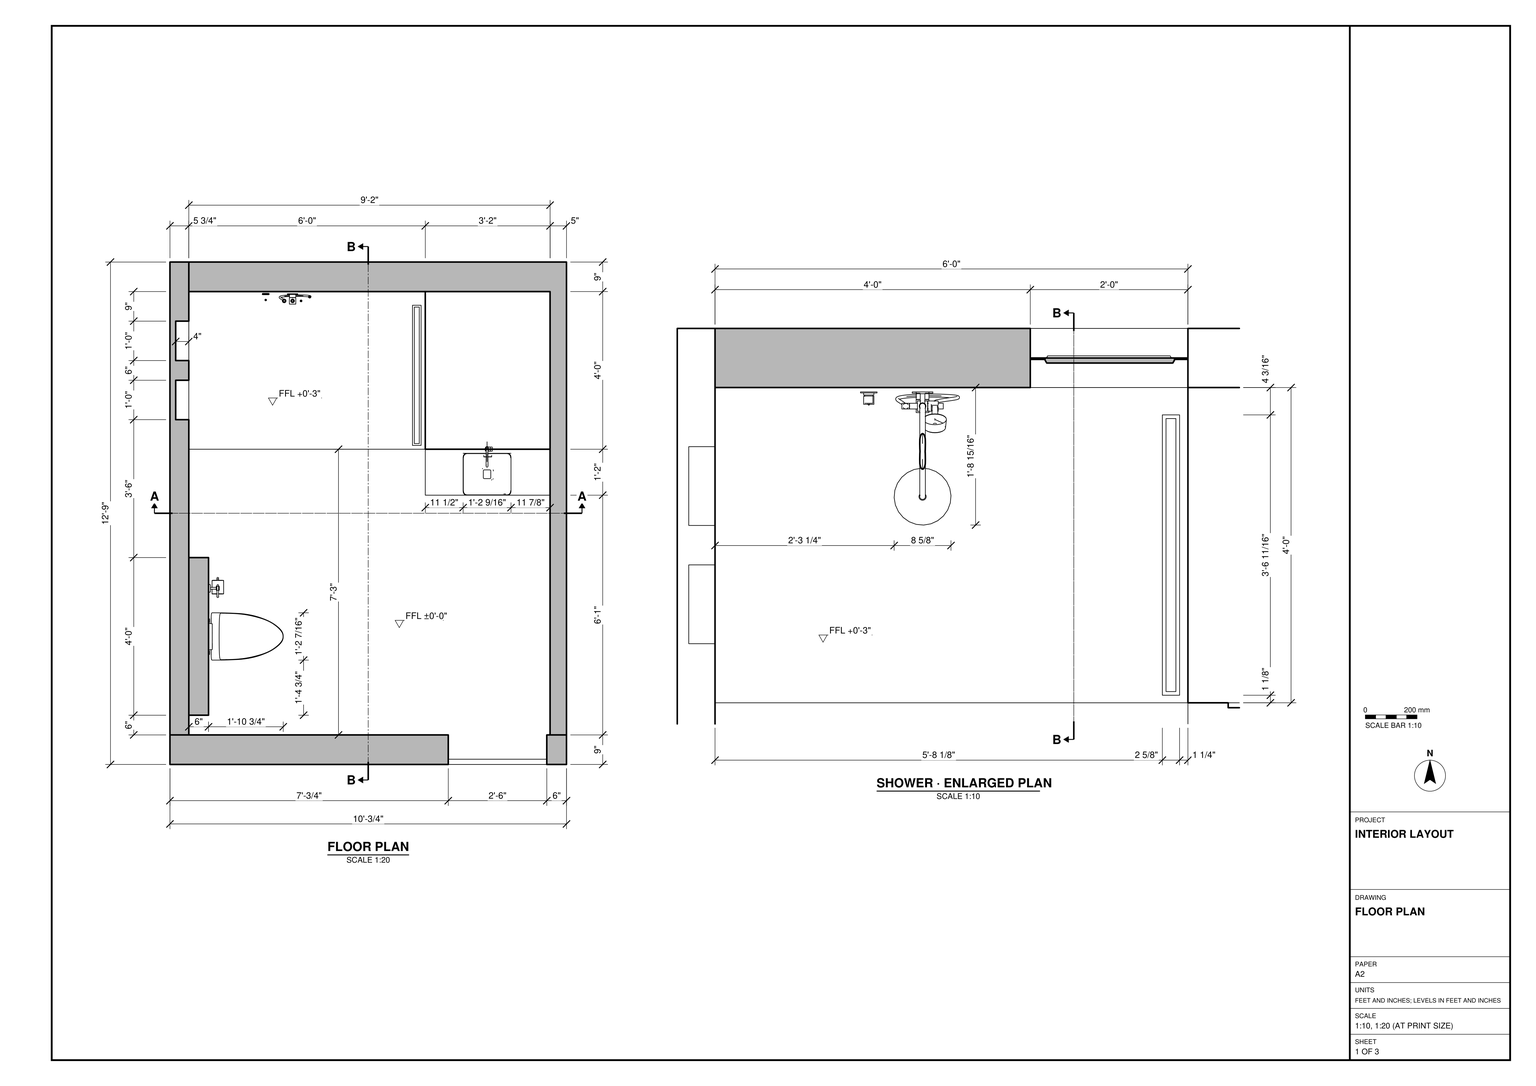
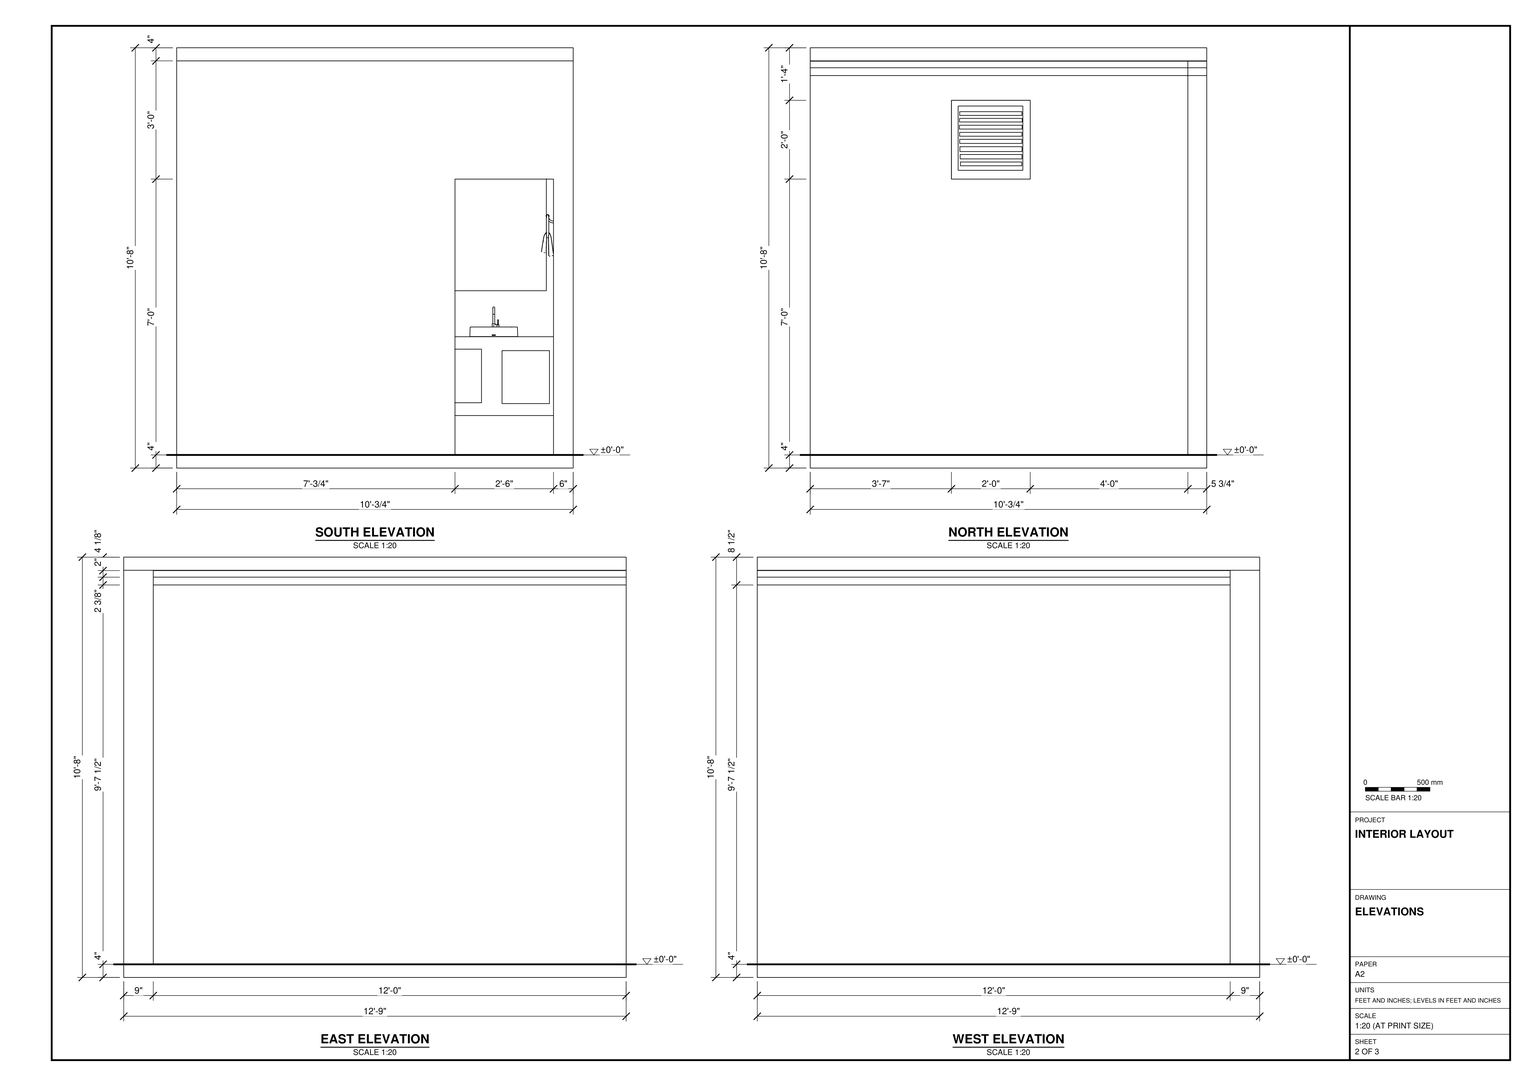
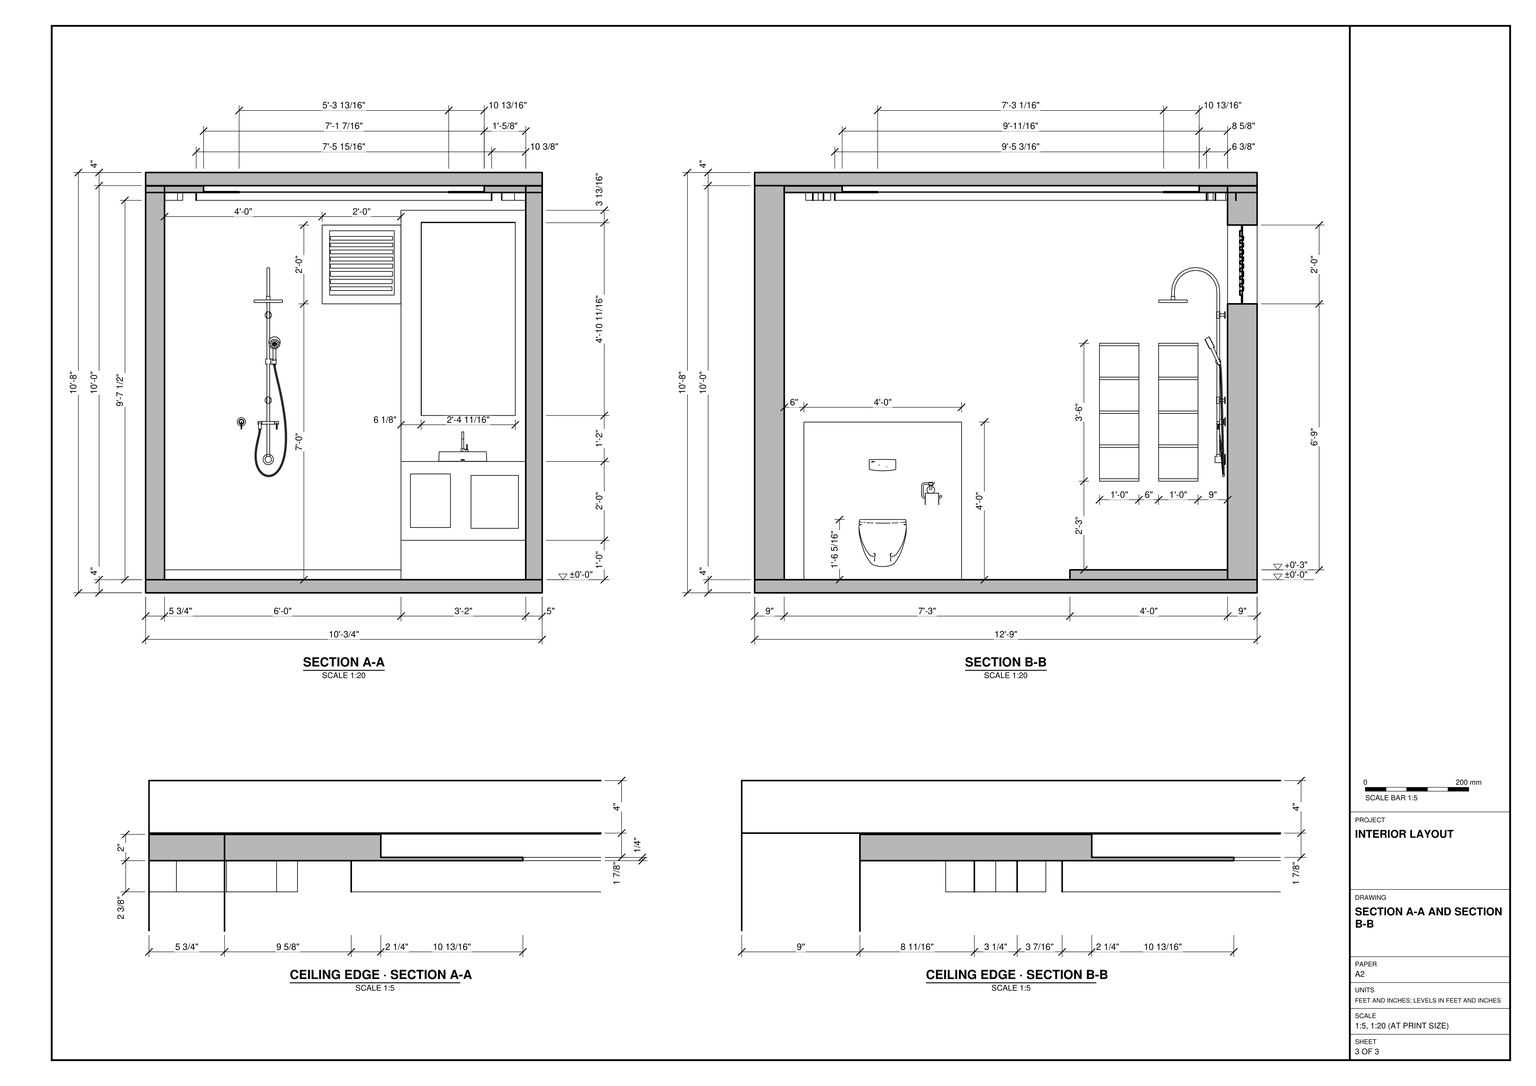
Build the bathroom in SketchUp from task_files/diagram_01.pdf. Work in feet and inches. The room shell measures 10'-3/4" east to west by 12'-9" north to south, with an overall height of 10'-8". Set the main finished floor at ±0'-0" and the raised shower floor at +0'-3". Use the floor plan for wall thicknesses and fixture positions, the elevations for openings, and the sections for vertical dimensions and the stepped ceiling edge.

Model the floor slab, perimeter walls and top slab. Leave the entry opening near the east end of the south wall and fit the square grille high in the north wall. In the northwest shower area, place the linear drain near the east edge, the shower fittings on the north wall and the two shelved recesses in the west wall. Position the vanity east of the shower, with its basin, faucet and tall mirror facing the entry. Mount the toilet on the low projecting wall south of the shower, with the flush plate above it.

Keep shell elements and each fixture, furniture or joinery piece in separate groups or components, and use components for repeated parts. Any decor or loose items shown may use suitable library components. Save one SketchUp model as output_files/bathroom_with_a_raised_shower_and_built_in_vanity.skp.

# SketchUp Ruby script. Lengths in inches.
U = 1.inch
M = Sketchup.active_model
def pt(a) = Geom::Point3d.new(a.map { |v| v * U })
def face(e, loops, mat)
  f = e.add_face(loops[0].map { |a| pt(a) })
  loops[1..].each { |l| e.add_face(l.map { |a| pt(a) }).erase! }
  f.material = f.back_material = mat if mat
  f
end
# faces: each face lists its corners as indices into pts; further lists are holes
def faces(e, pts, list, mat = nil) = list.each { |f| face(e, (f[0].is_a?(Array) ? f : [f]).map { |l| l.map { |i| pts[i] } }, mat) }
# xy, xz, yz: faces in a plane at the given z, y or x. An outline is a flat list of corners, or four numbers for a rectangle; further outlines are holes
def ring(l) = l.size == 4 ? [[l[0], l[1]], [l[2], l[1]], [l[2], l[3]], [l[0], l[3]]] : l.each_slice(2).to_a
def flat(e, list, mat, &to3) = list.each { |f| face(e, (f[0].is_a?(Array) ? f : [f]).map { |l| ring(l).map { |u, v| to3.(u, v) } }, mat) }
def xy(e, z, list, mat = nil) = flat(e, list, mat) { |x, y| [x, y, z] }
def xz(e, y, list, mat = nil) = flat(e, list, mat) { |x, z| [x, y, z] }
def yz(e, x, list, mat = nil) = flat(e, list, mat) { |y, z| [x, y, z] }
def lines(e, pts, list) = list.each { |a, b| e.add_line(pt(pts[a]), pt(pts[b])) }
# prism: a flat outline (further loops are holes) pulled along v
def prism(e, loops, v, mat = nil)
  f = face(e, loops, mat); d = Geom::Vector3d.new(v.map { |x| x * U })
  f.pushpull(f.normal.samedirection?(d) ? d.length : -d.length)
end
def box(e, o, s, mat = nil) = prism(e, [[o, [o[0] + s[0], o[1], o[2]], [o[0] + s[0], o[1] + s[1], o[2]], [o[0], o[1] + s[1], o[2]]]], [0, 0, s[2]], mat)
def at(x, y, z, deg = 0) = Geom::Transformation.translation(pt([x, y, z])) * Geom::Transformation.rotation(ORIGIN, Z_AXIS, deg.degrees)
def axes(o, x, y, z) = Geom::Transformation.new([*x, 0, *y, 0, *z, 0, *pt(o).to_a, 1])
def part(name) = M.definitions.add(name)
# library, detail: a bought-in or finely detailed component or shape, given as its bounding box
def library(name, o, s) = part(name).tap { |d| box(d.entities, o, s) }
def detail(e, o, s) = box(e.add_group.entities, o, s)
def put(e, d, t, mat = nil) = e.add_instance(d, t).tap { |i| i.material = mat if mat }
def group(e, t, mat = nil) = e.add_group.tap { |g| g.transformation = t; g.material = mat if mat }.entities
root = M.entities
M.materials.add("Black Ceramic").color = [0, 0, 0]
M.materials.add("[Basic Tile]").color = [148, 150, 147]
M.materials["[Basic Tile]"].alpha = 0.76
M.materials.add("[Chris_Hair]").color = [71, 76, 74]
M.materials.add("[Color A01]").color = [255, 204, 204]
M.materials.add("[Color C01]").color = [255, 229, 204]
M.materials.add("[Color J01]").color = [229, 204, 255]
M.materials.add("[Granite Light Gray]").color = [149, 148, 144]
M.materials.add("[Stone Vein Gray]").color = [165, 164, 164]
M.materials["[Stone Vein Gray]"].alpha = 0.69
M.materials.add("[Tile Travertine 2 inch]").color = [178, 175, 169]
M.materials.add("[Translucent Glass Sky Reflection]").color = [126, 138, 183]
M.materials["[Translucent Glass Sky Reflection]"].alpha = 0.52
M.materials.add("[Wood Cherry Original]").color = [152, 86, 42]
M.materials["[Wood Cherry Original]"].alpha = 0.95
M.materials.add("[Wood_ Floor]").color = [41, 29, 29]
M.materials.add("grille").color = [168, 171, 173]
M.materials.add("wire_127127127").color = [170, 170, 170]
c1 = library("3DGeom~7_Defintion",[-3164.19,2522.98,-2585.08],[573.68,1000,764.71])
c2 = library("Bathroom sink",[0,-15.75,0],[23.62,20.08,14.64])
c3 = part("Groupe\#1")
xy(c3.entities,0,[[[15.8,15.69,15.8,39.67,135.97,39.67,135.97,46.55,15.8,46.55,15.8,52.89,136.16,52.89,136.16,60.26,15.8,60.26,15.8,140.05,137,140.05,137,15.69],[15.83,94.34,135.28,103.79],[15.95,109.45,134.81,117.92],[15.9,80.03,135.59,88.03],[15.95,66.67,135.74,74.11],[16.02,26.56,135.61,33.79],[16.27,123.97,134.31,131.27]]],"[Chris_Hair]")
xy(c3.entities,2.02,[[[0,4.67,151.4,157.04],[14.22,15.69,138.58,140.05]]],"grille")
xy(c3.entities,2.81,[[[0,4.67,151.4,157.04],[15.83,94.34,135.28,103.79],[15.95,109.45,134.81,117.92],[15.9,80.03,135.59,88.03],[15.95,66.67,135.74,74.11],[15.67,52.89,136.16,60.26],[16.02,26.56,135.61,33.79],[16.27,123.97,134.31,131.27],[15.44,39.67,135.97,46.55]]],"grille")
xy(c3.entities,3.99,[[16.8,26.56,134.82,33.79],[16.23,39.67,135.18,46.55],[16.46,52.89,135.375,60.26],[16.74,66.67,134.95,74.11],[16.6875,80.03,134.8,88.03],
  [16.61,94.34,134.49,103.79],[16.74,109.45,134.02,117.92],[17.05,123.97,133.53,131.27]],"grille")
xz(c3.entities,4.67,[[0,2.02,151.4,2.81]],"grille")
xz(c3.entities,15.69,[[15.8,0,137,0,138.58,1.57,138.58,2.02,14.22,2.02,14.22,1.57]],"grille")
xz(c3.entities,26.56,[[16.02,0,16.02,3.2,16.8,3.99,134.82,3.99,135.61,3.2,135.61,0]],"grille")
xz(c3.entities,33.79,[[16.02,0,135.61,0,135.61,3.2,134.82,3.99,16.8,3.99,16.02,3.2]],"grille")
xz(c3.entities,39.67,[[15.44,0,15.44,3.2,16.23,3.99,135.18,3.99,135.97,3.2,135.97,0]],"grille")
xz(c3.entities,46.55,[[15.44,0,135.97,0,135.97,3.2,135.18,3.99,16.23,3.99,15.44,3.2]],"grille")
xz(c3.entities,52.89,[[15.67,0,15.67,3.2,16.46,3.99,135.375,3.99,136.16,3.2,136.16,0]],"grille")
xz(c3.entities,60.26,[[15.67,0,136.16,0,136.16,3.2,135.375,3.99,16.46,3.99,15.67,3.2]],"grille")
xz(c3.entities,66.67,[[15.95,0,15.95,3.2,16.74,3.99,134.95,3.99,135.74,3.2,135.74,0]],"grille")
xz(c3.entities,74.11,[[15.95,0,135.74,0,135.74,3.2,134.95,3.99,16.74,3.99,15.95,3.2]],"grille")
xz(c3.entities,80.03,[[15.9,0,15.9,3.2,16.6875,3.99,134.8,3.99,135.59,3.2,135.59,0]],"grille")
xz(c3.entities,88.03,[[15.9,0,135.59,0,135.59,3.2,134.8,3.99,16.6875,3.99,15.9,3.2]],"grille")
xz(c3.entities,94.34,[[15.83,0,15.83,3.2,16.61,3.99,134.49,3.99,135.28,3.2,135.28,0]],"grille")
xz(c3.entities,103.79,[[15.83,0,135.28,0,135.28,3.2,134.49,3.99,16.61,3.99,15.83,3.2]],"grille")
xz(c3.entities,109.45,[[15.95,0,15.95,3.2,16.74,3.99,134.02,3.99,134.81,3.2,134.81,0]],"grille")
xz(c3.entities,117.92,[[15.95,0,134.81,0,134.81,3.2,134.02,3.99,16.74,3.99,15.95,3.2]],"grille")
xz(c3.entities,123.97,[[16.27,0,16.27,3.2,17.05,3.99,133.53,3.99,134.31,3.2,134.31,0]],"grille")
xz(c3.entities,131.27,[[16.27,0,134.31,0,134.31,3.2,133.53,3.99,17.05,3.99,16.27,3.2]],"grille")
xz(c3.entities,140.05,[[15.8,0,14.22,1.57,14.22,2.02,138.58,2.02,138.58,1.57,137,0]],"grille")
xz(c3.entities,157.04,[[0,2.02,151.4,2.81]],"grille")
yz(c3.entities,0,[[4.67,2.02,157.04,2.81]],"grille")
yz(c3.entities,14.22,[[15.69,1.57,140.05,2.02]],"grille")
yz(c3.entities,15.44,[[39.67,0,46.55,3.2]],"grille")
yz(c3.entities,15.67,[[52.89,0,60.26,3.2]],"grille")
yz(c3.entities,15.83,[[94.34,0,103.79,3.2]],"grille")
yz(c3.entities,15.9,[[80.03,0,88.03,3.2]],"grille")
yz(c3.entities,15.95,[[66.67,0,74.11,3.2],[109.45,0,117.92,3.2]],"grille")
yz(c3.entities,16.02,[[26.56,0,33.79,3.2]],"grille")
yz(c3.entities,16.27,[[123.97,0,131.27,3.2]],"grille")
yz(c3.entities,134.31,[[123.97,0,131.27,3.2]],"grille")
yz(c3.entities,134.81,[[109.45,0,117.92,3.2]],"grille")
yz(c3.entities,135.28,[[94.34,0,103.79,3.2]],"grille")
yz(c3.entities,135.59,[[80.03,0,88.03,3.2]],"grille")
yz(c3.entities,135.61,[[26.56,0,33.79,3.2]],"grille")
yz(c3.entities,135.74,[[66.67,0,74.11,3.2]],"grille")
yz(c3.entities,135.97,[[39.67,0,46.55,3.2]],"grille")
yz(c3.entities,136.16,[[52.89,0,60.26,3.2]],"grille")
yz(c3.entities,138.58,[[15.69,1.57,140.05,2.02]],"grille")
yz(c3.entities,151.4,[[4.67,2.02,157.04,2.81]],"grille")
p = [[15.8,140.05,0],[15.8,60.26,0],[15.8,52.89,0],[15.8,46.55,0],[15.8,39.67,0],[15.8,15.69,0],
  [14.22,15.69,1.57],[14.22,140.05,1.57],[137,15.69,0],[137,140.05,0],[138.58,140.05,1.57],[138.58,15.69,1.57],
  [16.8,26.56,3.99],[16.8,33.79,3.99],[16.02,33.79,3.2],[16.02,26.56,3.2],[134.82,33.79,3.99],[134.82,26.56,3.99],
  [135.61,26.56,3.2],[135.61,33.79,3.2],[16.23,39.67,3.99],[16.23,46.55,3.99],[15.44,46.55,3.2],[15.44,39.67,3.2],
  [135.18,46.55,3.99],[135.18,39.67,3.99],[135.97,39.67,3.2],[135.97,46.55,3.2],[16.46,52.89,3.99],[16.46,60.26,3.99],
  [15.67,60.26,3.2],[15.67,52.89,3.2],[135.375,60.26,3.99],[135.375,52.89,3.99],[136.16,52.89,3.2],[136.16,60.26,3.2],
  [16.74,66.67,3.99],[16.74,74.11,3.99],[15.95,74.11,3.2],[15.95,66.67,3.2],[134.95,74.11,3.99],[134.95,66.67,3.99],
  [135.74,66.67,3.2],[135.74,74.11,3.2],[16.6875,80.03,3.99],[16.6875,88.03,3.99],[15.9,88.03,3.2],[15.9,80.03,3.2],
  [134.8,88.03,3.99],[134.8,80.03,3.99],[135.59,80.03,3.2],[135.59,88.03,3.2],[16.61,94.34,3.99],[16.61,103.79,3.99],
  [15.83,103.79,3.2],[15.83,94.34,3.2],[134.49,103.79,3.99],[134.49,94.34,3.99],[135.28,94.34,3.2],[135.28,103.79,3.2],
  [16.74,109.45,3.99],[16.74,117.92,3.99],[15.95,117.92,3.2],[15.95,109.45,3.2],[134.02,117.92,3.99],[134.02,109.45,3.99],
  [134.81,109.45,3.2],[134.81,117.92,3.2],[17.05,123.97,3.99],[17.05,131.27,3.99],[16.27,131.27,3.2],[16.27,123.97,3.2],
  [133.53,131.27,3.99],[133.53,123.97,3.99],[134.31,123.97,3.2],[134.31,131.27,3.2]]
faces(c3.entities,p,[[0,1,2,3,4,5,6,7],[8,9,10,11]],"[Chris_Hair]")
faces(c3.entities,p,[[12,13,14,15],[16,17,18,19],[20,21,22,23],[24,25,26,27],[28,29,30,31],[32,33,34,35],[36,37,38,39],[40,41,42,43],
  [44,45,46,47],[48,49,50,51],[52,53,54,55],[56,57,58,59],[60,61,62,63],[64,65,66,67],[68,69,70,71],[72,73,74,75]],"grille")
lines(c3.entities,p,[[0,5]])
c4 = part("grille")
put(c4.entities,c3,axes([0,66.92,74.4],[1,0,0],[0,0,-1],[0,1,0]))
c5 = part("d3")
xy(c5.entities,0,[[0,0,36,1.6]],"[Wood_ Floor]")
xy(c5.entities,72,[[0,0,36,1.6]],"[Wood_ Floor]")
yz(c5.entities,0,[[0,0,1.6,72]],"[Wood_ Floor]")
yz(c5.entities,36,[[0,0,1.6,72]],"[Wood_ Floor]")
c6 = part("Group\#5")
box(c6.entities,[0,0,0],[4,12,0.75])
c7 = library("3DGeom~3_Defintion",[-3150.4,3815.04,-609.52],[129.67,427.45,1000])
c8 = library("Group\#7",[0,0,0],[22.75,14.41,14.34])
c9 = library("Group\#8",[0,0,0],[4.69,6.89,12.89])
c10 = library("Group\#17",[0,0,0],[15.06,20.27,63.73])
put(root,c1,axes([37.25,36.15,5.34],[0.00806,0,0],[0,0,0.00806],[0,-0.00806,0]),"wire_127127127")
put(root,c2,axes([89.27,94.75,40.05],[0.61738,0,0],[0,0.80984,0],[0,0,0.61738]))
put(root,c4,axes([53.75,129.43,101.01],[0.15835,0,0],[0,0.27355,0],[0,0,0.15741]))
put(root,c5,axes([84.75,0,4],[0.83333,0,0],[0,1,0],[0,0,1.16667]))
g1 = group(root,at(0.75,9,0))
xy(g1,0,[[-0.75,-9,120,144]])
xy(g1,4,[[-0.75,-9,120,144]],"[Basic Tile]")
xz(g1,-9,[[-0.75,0,120,4]],"[Color A01]")
xz(g1,144,[[-0.75,0,120,4]],"[Color A01]")
yz(g1,-0.75,[[-9,0,144,4]],"[Color A01]")
yz(g1,120,[[-9,0,144,4]],"[Color A01]")
g2 = group(root,at(5.75,9,4))
xy(g2,0,[[110,0,110,135,0,135,0,144,115,144,115,0]])
xy(g2,84,[[48,135,72,144]],"[Tile Travertine 2 inch]")
xy(g2,108,[[48,135,72,144]],"[Tile Travertine 2 inch]")
xy(g2,120,[[110,0,115,0,115,144,0,144,0,135,110,135]])
xz(g2,0,[[110,0,115,120]])
xz(g2,135,[[[0,0,110,120],[48,84,72,108]]],"[Tile Travertine 2 inch]")
xz(g2,144,[[[0,0,115,120],[48,84,72,108]]],"[Color C01]")
yz(g2,0,[[135,0,144,120]])
yz(g2,48,[[135,84,144,108]],"[Tile Travertine 2 inch]")
yz(g2,72,[[135,84,144,108]],"[Tile Travertine 2 inch]")
yz(g2,110,[[0,0,135,120]],"[Tile Travertine 2 inch]")
yz(g2,115,[[0,0,144,120]],"[Color C01]")
g3 = group(root,at(0.75,9,4))
xy(g3,0,[[-0.75,0,5,144]])
xy(g3,30,[[1,96,5,108],[1,114,5,126]])
xy(g3,72,[[1,96,5,108],[1,114,5,126]])
xy(g3,120,[[-0.75,0,5,144]])
xz(g3,0,[[-0.75,0,5,120]])
xz(g3,96,[[1,30,5,72]],"[Basic Tile]")
xz(g3,108,[[1,30,5,72]],"[Basic Tile]")
xz(g3,114,[[1,30,5,72]],"[Basic Tile]")
xz(g3,126,[[1,30,5,72]],"[Basic Tile]")
xz(g3,144,[[-0.75,0,5,120]],"[Color C01]")
yz(g3,-0.75,[[0,0,144,120]],"[Color C01]")
yz(g3,1,[[96,30,108,72],[114,30,126,72]],"[Basic Tile]")
yz(g3,5,[[[0,0,144,120],[96,30,108,72],[114,30,126,72]]],"[Tile Travertine 2 inch]")
g4 = group(root,at(77.75,96,4))
xy(g4,0,[[0,0,38,48]])
xy(g4,12,[[0,-14,38,0]])
xy(g4,15.64,[[21.33,-14,35.76,-1]],"[Wood Cherry Original]")
xy(g4,15.9,[[2.88,-14,15.07,-1]],"[Wood Cherry Original]")
xy(g4,31.76,[[21.33,-14,35.76,-1]])
xy(g4,32.21,[[2.88,-14,15.07,-1]])
xy(g4,36,[[0,-14,38,0]],"[Granite Light Gray]")
xy(g4,50.01,[[6.13,-0.75,34.82,0]])
xy(g4,108.88,[[6.13,-0.75,34.82,0]])
xy(g4,112.5,[[0,0,38,48]])
xz(g4,-14,[[[0,12,38,36],[21.33,15.64,35.76,31.76],[2.88,15.9,15.07,32.21]]],"[Wood Cherry Original]")
xz(g4,-1,[[21.33,15.64,35.76,31.76],[2.88,15.9,15.07,32.21]],"[Wood Cherry Original]")
xz(g4,0,[[0,0,38,12],[[0,36,38,112.5],[6.13,50.01,34.82,108.88]]],"[Basic Tile]")
xz(g4,48,[[0,0,38,112.5]])
yz(g4,0,[[0,0,48,112.5]],"[Tile Travertine 2 inch]")
yz(g4,0,[[-14,12,0,36]],"[Wood Cherry Original]")
yz(g4,2.88,[[-14,15.9,-1,32.21]],"[Wood Cherry Original]")
yz(g4,6.13,[[-0.75,50.01,0,108.88]])
yz(g4,15.07,[[-14,15.9,-1,32.21]],"[Wood Cherry Original]")
yz(g4,21.33,[[-14,15.64,-1,31.76]],"[Wood Cherry Original]")
yz(g4,34.82,[[-0.75,50.01,0,108.88]])
yz(g4,35.76,[[-14,15.64,-1,31.76]],"[Wood Cherry Original]")
yz(g4,38,[[0,0,48,0,48,112.5,0,112.5,0,36,-14,36,-14,12,0,12]])
g5 = group(g4,at(6.22,-0.75,50.01),"[Translucent Glass Sky Reflection]")
xz(g5,0,[[0,0,28.6,58.6875]])
put(root,c6,at(1.75,105,34))
put(root,c6,at(1.75,105,44.3125))
put(root,c6,at(1.75,105,54.625))
put(root,c6,at(1.75,105,64.9375))
put(root,c6,at(1.75,105,75.25))
put(root,c6,at(1.75,123,34))
put(root,c6,at(1.75,123,64.9375))
put(root,c6,at(1.75,123,75.25))
put(root,c6,at(1.75,123,44.3125))
put(root,c6,at(1.75,123,54.625))
g6 = group(root,at(5.75,15,4))
xy(g6,0,[[0,0,6,48]])
xy(g6,48,[[0,0,6,48]],"[Basic Tile]")
xz(g6,0,[[0,0,6,48]],"[Basic Tile]")
xz(g6,48,[[0,0,6,48]],"[Basic Tile]")
yz(g6,0,[[0,0,48,48]])
yz(g6,6,[[0,0,48,48]],"[Basic Tile]")
g7 = group(root,at(37.33,38.05,6.33))
put(g7,c7,axes([0,0,0],[0.00809,0,0],[0,0,0.00809],[0,-0.00809,0]),"Black Ceramic")
put(root,c8,at(11.75,31.78,8))
put(root,c9,at(115.75,75.93,64.33,-180))
put(root,c10,at(27.9,123.0625,35.35))
g8 = group(root,at(0.75,9,124))
xy(g8,0,[[-0.75,-9,120,144]])
xy(g8,4,[[-0.75,-9,120,144]],"[Color C01]")
xz(g8,-9,[[-0.75,0,120,4]],"[Color A01]")
xz(g8,144,[[-0.75,0,120,4]],"[Color A01]")
yz(g8,-0.75,[[-9,0,144,4]],"[Color A01]")
yz(g8,120,[[-9,0,144,4]],"[Color A01]")
g9 = group(root,at(0,9,106.4))
g10 = group(g9,at(0.75,0,15.5))
xy(g10,0,[[[-0.75,0,120,144],[27.71,28.46,91.54,115.54]]])
xy(g10,0.25,[[[16.9,17.65,102.35,126.35],[27.71,28.46,91.54,115.54]]])
xy(g10,2,[[[-0.75,0,120,144],[16.9,17.65,102.35,126.35]]])
xz(g10,0,[[-0.75,0,120,2]])
xz(g10,17.65,[[16.9,0.25,102.35,2]])
xz(g10,28.46,[[27.71,0,91.54,0.25]])
xz(g10,115.54,[[27.71,0,91.54,0.25]])
xz(g10,126.35,[[16.9,0.25,102.35,2]])
xz(g10,144,[[-0.75,0,120,2]])
yz(g10,-0.75,[[0,0,144,2]])
yz(g10,16.9,[[17.65,0.25,126.35,2]])
yz(g10,27.71,[[28.46,0,115.54,0.25]])
yz(g10,91.54,[[28.46,0,115.54,0.25]])
yz(g10,102.35,[[17.65,0.25,126.35,2]])
yz(g10,120,[[0,0,144,2]])
g11 = group(g9,at(0.75,0,13.5))
xy(g11,-0.375,[[65.49,10.21,65.62,10.34,61.81,14.15,61.68,14.02]])
xy(g11,2,[[[-0.75,0,120,144],[14.64,15.39,104.61,128.61],[111.4,124.46,107.59,128.27,111.4,132.08,115.21,128.27],[7.31,6.53,3.5,10.34,7.31,14.15,11.12,10.34],[111.25,6.53,107.43,10.34,111.25,14.15,115.06,10.34],[6.74,125.25,2.93,129.07,6.74,132.88,10.55,129.07],[111.59,71.27,107.77,75.09,111.59,78.9,115.4,75.09],[5.15,73.08,1.34,76.89,5.15,80.7,8.96,76.89],[61.81,6.53,58,10.34,61.81,14.15,65.62,10.34],[58.94,130.6,55.12,134.41,58.94,138.23,62.75,134.41]]])
xz(g11,0,[[-0.75,-0.375,120,2]])
xz(g11,15.39,[[14.64,-0.375,104.61,2]])
xz(g11,128.61,[[14.64,-0.375,104.61,2]])
xz(g11,144,[[-0.75,-0.375,120,2]])
yz(g11,-0.75,[[0,-0.375,144,2]])
yz(g11,14.64,[[15.39,-0.375,128.61,2]])
yz(g11,104.61,[[15.39,-0.375,128.61,2]])
yz(g11,120,[[0,-0.375,144,2]])
p = [[3.5,10.34,-0.375],[3.5,10.34,2],[7.31,6.53,2],[7.31,6.53,-0.375],[11.12,10.34,2],[11.12,10.34,-0.375],
  [58,10.34,-0.375],[58,10.34,2],[61.81,6.53,2],[61.81,6.53,-0.375],[111.25,6.53,-0.375],[107.43,10.34,-0.375],
  [107.43,10.34,2],[111.25,6.53,2],[115.06,10.34,-0.375],[115.06,10.34,2],[7.31,14.15,-0.375],[7.31,14.15,2],
  [61.81,14.15,-0.375],[61.81,14.15,2],[61.68,14.02,-0.375],[65.62,10.34,-0.375],[65.62,10.34,2],[111.25,14.15,-0.375],
  [111.25,14.15,2],[111.59,71.27,-0.375],[107.77,75.09,-0.375],[107.77,75.09,2],[111.59,71.27,2],[115.4,75.09,-0.375],
  [115.4,75.09,2],[5.15,73.08,-0.375],[1.34,76.89,-0.375],[1.34,76.89,2],[5.15,73.08,2],[8.96,76.89,-0.375],
  [8.96,76.89,2],[111.59,78.9,-0.375],[111.59,78.9,2],[5.15,80.7,-0.375],[5.15,80.7,2],[111.4,124.46,-0.375],
  [107.59,128.27,-0.375],[107.59,128.27,2],[111.4,124.46,2],[115.21,128.27,-0.375],[115.21,128.27,2],[6.74,125.25,-0.375],
  [2.93,129.07,-0.375],[2.93,129.07,2],[6.74,125.25,2],[10.55,129.07,-0.375],[10.55,129.07,2],[111.4,132.08,-0.375],
  [111.4,132.08,2],[6.74,132.88,-0.375],[6.74,132.88,2],[58.94,130.6,-0.375],[55.12,134.41,-0.375],[55.12,134.41,2],
  [58.94,130.6,2],[62.75,134.41,-0.375],[62.75,134.41,2],[58.94,138.23,-0.375],[58.94,138.23,2],[65.62,10.34,-13.5],
  [65.49,10.21,-13.5]]
faces(g11,p,[[0,1,2,3],[3,2,4,5],[6,7,8,9],[10,11,12,13],[14,10,13,15],[16,17,1,0],[5,4,17,16],[18,19,7,6,20],
  [21,22,19,18],[11,23,24,12],[23,14,15,24],[25,26,27,28],[29,25,28,30],[31,32,33,34],[35,31,34,36],[26,37,38,27],
  [37,29,30,38],[32,39,40,33],[39,35,36,40],[41,42,43,44],[45,41,44,46],[47,48,49,50],[51,47,50,52],[42,53,54,43],
  [53,45,46,54],[48,55,56,49],[55,51,52,56],[57,58,59,60],[61,57,60,62],[58,63,64,59],[63,61,62,64]])
lines(g11,p,[[65,66]])
g12 = group(root,at(0,0,4))
xy(g12,0,[[0,0,84.75,9],[114.75,0,120.75,9]])
xy(g12,84,[[84.75,0,114.75,9]],"[Color J01]")
xy(g12,120,[[0,0,120.75,9]])
xz(g12,0,[[0,0,84.75,0,84.75,84,114.75,84,114.75,0,120.75,0,120.75,120,0,120]],"[Color C01]")
xz(g12,9,[[0,0,0,120,120.75,120,120.75,0,114.75,0,114.75,84,84.75,84,84.75,0]],"[Tile Travertine 2 inch]")
yz(g12,0,[[0,0,9,120]],"[Color C01]")
yz(g12,84.75,[[0,0,9,84]],"[Color J01]")
yz(g12,114.75,[[0,0,9,84]],"[Color J01]")
yz(g12,120.75,[[0,0,9,120]],"[Color C01]")
g13 = group(root,at(5.75,96,4))
xy(g13,0,[[0,0,72,48]])
xy(g13,2.4375,[[[68.1,1.15,70.73,43.84],[68.66,1.71,70.17,43.28]],[68.66,1.71,70.17,43.28]],"Black Ceramic")
xy(g13,3,[[[0,0,72,48],[68.1,1.15,70.73,43.84]]],"[Stone Vein Gray]")
xz(g13,0,[[0,0,72,3]],"[Stone Vein Gray]")
xz(g13,1.15,[[68.1,2.4375,70.73,3]],"[Stone Vein Gray]")
xz(g13,43.84,[[68.1,2.4375,70.73,3]],"[Stone Vein Gray]")
xz(g13,48,[[0,0,72,3]])
yz(g13,0,[[0,0,48,3]])
yz(g13,68.1,[[1.15,2.4375,43.84,3]],"[Stone Vein Gray]")
yz(g13,70.73,[[1.15,2.4375,43.84,3]],"[Stone Vein Gray]")
yz(g13,72,[[0,0,48,3]])
p = [[72,0,36],[72,0,3]]
lines(g13,p,[[0,1]])
